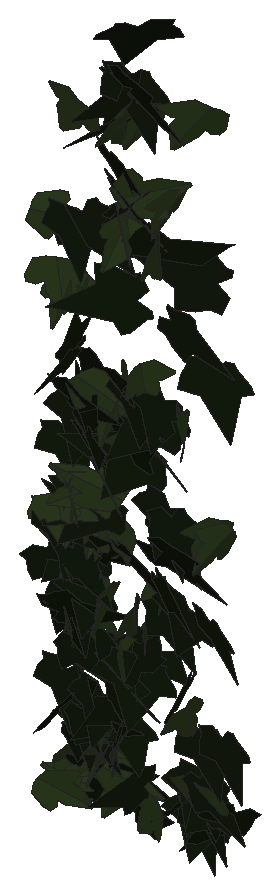
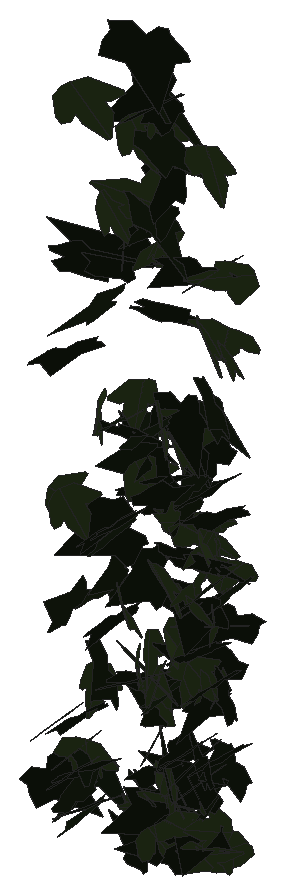
# SketchUp Ruby script. Lengths in inches.
U = 1.inch
M = Sketchup.active_model
def pt(a) = Geom::Point3d.new(a.map { |v| v * U })
def face(e, loops, mat)
  f = e.add_face(loops[0].map { |a| pt(a) })
  loops[1..].each { |l| e.add_face(l.map { |a| pt(a) }).erase! }
  f.material = f.back_material = mat if mat
  f
end
# faces: each face lists its corners as indices into pts; further lists are holes
def faces(e, pts, list, mat = nil) = list.each { |f| face(e, (f[0].is_a?(Array) ? f : [f]).map { |l| l.map { |i| pts[i] } }, mat) }
# xy, xz, yz: faces in a plane at the given z, y or x. An outline is a flat list of corners, or four numbers for a rectangle; further outlines are holes
def ring(l) = l.size == 4 ? [[l[0], l[1]], [l[2], l[1]], [l[2], l[3]], [l[0], l[3]]] : l.each_slice(2).to_a
def flat(e, list, mat, &to3) = list.each { |f| face(e, (f[0].is_a?(Array) ? f : [f]).map { |l| ring(l).map { |u, v| to3.(u, v) } }, mat) }
def xy(e, z, list, mat = nil) = flat(e, list, mat) { |x, y| [x, y, z] }
def xz(e, y, list, mat = nil) = flat(e, list, mat) { |x, z| [x, y, z] }
def yz(e, x, list, mat = nil) = flat(e, list, mat) { |y, z| [x, y, z] }
def lines(e, pts, list) = list.each { |a, b| e.add_line(pt(pts[a]), pt(pts[b])) }
# prism: a flat outline (further loops are holes) pulled along v
def prism(e, loops, v, mat = nil)
  f = face(e, loops, mat); d = Geom::Vector3d.new(v.map { |x| x * U })
  f.pushpull(f.normal.samedirection?(d) ? d.length : -d.length)
end
def box(e, o, s, mat = nil) = prism(e, [[o, [o[0] + s[0], o[1], o[2]], [o[0] + s[0], o[1] + s[1], o[2]], [o[0], o[1] + s[1], o[2]]]], [0, 0, s[2]], mat)
def at(x, y, z, deg = 0) = Geom::Transformation.translation(pt([x, y, z])) * Geom::Transformation.rotation(ORIGIN, Z_AXIS, deg.degrees)
def axes(o, x, y, z) = Geom::Transformation.new([*x, 0, *y, 0, *z, 0, *pt(o).to_a, 1])
def part(name) = M.definitions.add(name)
# library, detail: a bought-in or finely detailed component or shape, given as its bounding box
def library(name, o, s) = part(name).tap { |d| box(d.entities, o, s) }
def detail(e, o, s) = box(e.add_group.entities, o, s)
def put(e, d, t, mat = nil) = e.add_instance(d, t).tap { |i| i.material = mat if mat }
def group(e, t, mat = nil) = e.add_group.tap { |g| g.transformation = t; g.material = mat if mat }.entities
root = M.entities
M.materials.add("1026 AP 7946 SUNNY SIDE UP").color = [254, 231, 186]
M.materials.add("efeu1").color = [18, 25, 13]
M.materials.add("efeu2").color = [43, 57, 29]
c1 = part("ivyleaf_9")
p = [[1.54,2.16,1.25],[1.36,2.04,1.19],[-0.21,0.99,0.68],[-0.71,1.11,0.82],[-0.85,0.86,0.67],[-0.8,0.17,0.21],
  [-0.9,-0.01,0.1],[-0.67,-0.16,-0.02],[-0.08,-0.08,-0.05],[-0.03,-0.6,-0.4],[0.65,-0.88,-0.66],[0.83,-0.6,-0.49],
  [1.29,-0.42,-0.43],[1.8125,-0.07,-0.26],[1.21,0.44,0.15]]
faces(c1.entities,p,[[0,1,2,3,4,5,6,7,8,9,10,11,12,13,14]],"efeu1")
c2 = part("ivyleaf_10")
p = [[0,0.5,-0.03],[-0.0625,2.02,-0.43],[-0.19,2.01,-0.46],[-0.54,1.05,-0.29],[-0.52,0.625,-0.18],[-0.83,0.76,-0.28],
  [-1.16,0.64,-0.33],[-1.15,0.33,-0.24],[-0.77,-0.39,0.02],[-0.3,-0.51,0.16],[0.04,-0.48,0.23],[-0.02,2.01,-0.4375],
  [-0.06,2.01,-0.43],[0.04,-0.49,0.23],[0.67,-0.49,0.14],[1.38,0.36,-0.2],[1.375,0.51,-0.24],[0.81,0.65,-0.19],
  [0.62,0.59,-0.15],[0.6,1.09,-0.28],[0.5,1.23,-0.31]]
faces(c2.entities,p,[[0,1,2,3,4,5,6,7,8,9,10],[11,12,0,13,14,15,16,17,18,19,20]],"efeu2")
put(root,c1,axes([98.92,212.57,271.74],[0.07867,-0.26542,0.05597],[0.00956,-0.05567,-0.27854],[0.42638,0.05022,-0.00408]),"1026 AP 7946 SUNNY SIDE UP")
put(root,c1,axes([98.86,212.73,270.37],[0.00768,-0.04283,-0.2465],[0.3907,-0.03878,0.01205],[-0.06836,-0.22644,0.0412]),"1026 AP 7946 SUNNY SIDE UP")
put(root,c1,axes([99,212.74,269.39],[-0.03645,-0.26385,0.03472],[0.00036,-0.03535,-0.27305],[0.41855,-0.02295,0.00326]),"1026 AP 7946 SUNNY SIDE UP")
put(root,c2,axes([99.3125,212.57,277.98],[-0.37981,0.0743,0.14082],[-0.22478,0.01308,-0.25071],[-0.12044,-0.25872,0.02385]),"1026 AP 7946 SUNNY SIDE UP")
put(root,c1,axes([98.98,212.42,271.33],[-0.01322,-0.0951,-0.23583],[0.03641,0.21799,-0.0991],[0.40373,-0.02277,0.00122]),"1026 AP 7946 SUNNY SIDE UP")
put(root,c2,axes([98.875,212.42,276.33],[-0.04788,-0.07198,-0.2635],[0.37477,0.11735,-0.06243],[0.21843,-0.21712,0.04937]),"1026 AP 7946 SUNNY SIDE UP")
put(root,c1,axes([99,212.88,270.51],[0.01475,-0.27299,0.01382],[-0.00066,-0.01499,-0.28148],[0.42989,0.00934,-0.00091]),"1026 AP 7946 SUNNY SIDE UP")
put(root,c2,axes([99.1,212.57,270.43],[-0.15573,0.20855,-0.03662],[0.01063,-0.03755,-0.24424],[-0.35937,-0.09148,0.00865]),"1026 AP 7946 SUNNY SIDE UP")
put(root,c1,axes([99.23,212.52,274.39],[0.03624,0.127,0.23148],[0.01277,0.21493,-0.13399],[-0.42306,0.01737,0.01579]),"1026 AP 7946 SUNNY SIDE UP")
put(root,c1,axes([99.18,212.2,269.04],[-0.11239,0.14177,-0.19948],[-0.14207,0.16857,0.16984],[0.37387,0.10667,0.00457]),"1026 AP 7946 SUNNY SIDE UP")
put(root,c1,axes([99.05,212.72,272.94],[-0.07188,-0.22594,-0.06483],[0.03407,0.05481,-0.24513],[0.39435,-0.04592,0.00936]),"1026 AP 7946 SUNNY SIDE UP")
put(root,c2,axes([99.03,212.49,275.49],[0.40704,0.0632,0.06254],[0.10403,-0.00744,-0.26451],[-0.10122,0.24649,-0.02035]),"1026 AP 7946 SUNNY SIDE UP")
put(root,c2,axes([99.1,212.5,275.24],[0.30867,-0.16116,0.08469],[0.08643,-0.06478,-0.2606],[0.29391,0.18831,-0.01231]),"1026 AP 7946 SUNNY SIDE UP")
put(root,c2,axes([99.14,212.65,271.32],[-0.04199,0.10192,-0.22427],[-0.01397,-0.21223,-0.11177],[-0.39724,-0.00331,0.02764]),"1026 AP 7946 SUNNY SIDE UP")
put(root,c2,axes([99.38,212.73,267.82],[0.08322,0.11882,0.19662],[-0.24675,-0.12093,0.12467],[0.27453,-0.14471,0.05245]),"1026 AP 7946 SUNNY SIDE UP")
put(root,c1,axes([99.24,212.87,271.3],[-0.32905,-0.15842,0.09008],[0.00645,-0.13898,-0.24755],[0.28514,-0.17967,0.10956]),"1026 AP 7946 SUNNY SIDE UP")
put(root,c1,axes([99.31,212.53,274.33],[-0.25359,0.14222,-0.14828],[0.14119,-0.11509,-0.22122],[-0.30842,-0.16963,0.02065]),"1026 AP 7946 SUNNY SIDE UP")
put(root,c2,axes([99.125,212.53,268.2],[0.03368,-0.07345,0.23194],[0.03077,0.21824,0.08013],[-0.38865,0.01091,0.02644]),"1026 AP 7946 SUNNY SIDE UP")
put(root,c1,axes([99.36,212.88,271.6],[-0.03499,-0.27639,0.02424],[-0.00437,0.0254,0.28576],[-0.43636,0.02191,-0.00481]),"1026 AP 7946 SUNNY SIDE UP")
put(root,c1,axes([99.14,212.89,273.28],[-0.08545,-0.26215,0.09747],[-0.01725,-0.09582,-0.27623],[0.43869,-0.05483,0.00812]),"1026 AP 7946 SUNNY SIDE UP")
put(root,c2,axes([99.11,212.41,272.04],[0.35837,0.11994,0.04029],[0.0667,0.0037,-0.25932],[-0.20188,0.21414,-0.01416]),"1026 AP 7946 SUNNY SIDE UP")
put(root,c2,axes([99.06,212.31,267.91],[0.14805,0.09457,0.22014],[0.16656,0.18134,-0.13211],[-0.34412,0.12846,0.03076]),"1026 AP 7946 SUNNY SIDE UP")
put(root,c2,axes([99.15,212.54,267.93],[-0.1139,-0.11677,-0.19195],[0.19081,0.13878,-0.14107],[0.30651,-0.12979,0.01649]),"1026 AP 7946 SUNNY SIDE UP")
put(root,c2,axes([99.33,212.77,270.56],[-0.04162,-0.18797,0.12553],[-0.01659,-0.1194,-0.20454],[0.37794,-0.02594,0.00485]),"1026 AP 7946 SUNNY SIDE UP")
put(root,c2,axes([99.29,212.63,272.46],[0.08752,-0.21726,0.08136],[0.03333,-0.07636,-0.24011],[0.39091,0.05515,0.00226]),"1026 AP 7946 SUNNY SIDE UP")
put(root,c1,axes([99.47,212.72,272.12],[-0.36186,-0.07658,0.07247],[-0.08933,-0.05464,-0.24079],[0.15006,-0.21719,0.03142]),"1026 AP 7946 SUNNY SIDE UP")
put(root,c1,axes([99.16,212.8,269.08],[-0.02107,0.07026,0.23407],[0.0508,-0.21567,0.07333],[0.38503,0.0323,0.00313]),"1026 AP 7946 SUNNY SIDE UP")
put(root,c2,axes([99.26,212.49,272.22],[-0.15565,0.21968,-0.04486],[0.01506,-0.04478,-0.25529],[-0.38028,-0.09169,0.00825]),"1026 AP 7946 SUNNY SIDE UP")
put(root,c2,axes([99.36,212.56,275.41],[0.24966,-0.21134,-0.03509],[-0.03837,0.02083,-0.27527],[0.36032,0.14865,-0.005]),"1026 AP 7946 SUNNY SIDE UP")
put(root,c1,axes([99.21,212.56,268.68],[0.25063,-0.15497,-0.12351],[-0.13651,0.07993,-0.22801],[0.29595,0.1681,-0.00057]),"1026 AP 7946 SUNNY SIDE UP")
put(root,c2,axes([99.33,212.66,272.34],[0.06516,0.18271,-0.15873],[-0.04183,-0.1487,-0.20188],[-0.3998,0.04534,-0.00475]),"1026 AP 7946 SUNNY SIDE UP")
put(root,c1,axes([99.28,212.56,270.07],[0.05915,-0.14534,-0.19283],[-0.10046,0.16852,-0.15716],[0.37724,0.06767,-0.01162]),"1026 AP 7946 SUNNY SIDE UP")
put(root,c1,axes([99.36,212.64,268.24],[0.2761,0.14314,-0.04618],[-0.04147,-0.04022,-0.23205],[-0.25132,0.16389,-0.01245]),"1026 AP 7946 SUNNY SIDE UP")
put(root,c2,axes([99.41,212.72,270.45],[-0.35828,0.08586,-0.01357],[0.00713,-0.02609,-0.2431],[-0.14745,-0.20989,0.02121]),"1026 AP 7946 SUNNY SIDE UP")
put(root,c1,axes([99.39,212.65,271.53],[0.34596,0.06539,-0.11656],[-0.16857,-0.04885,-0.2293],[-0.13639,0.22625,-0.01225]),"1026 AP 7946 SUNNY SIDE UP")
put(root,c1,axes([99.27,212.53,276.28],[-0.00853,-0.26095,0.05202],[-0.00284,-0.05197,-0.28015],[0.45168,-0.00526,-0.00078]),"1026 AP 7946 SUNNY SIDE UP")
put(root,c2,axes([99.4,212.76,271.79],[0.06635,0.20411,-0.11197],[-0.02304,-0.10656,-0.22389],[-0.39073,0.04094,-0.00581]),"1026 AP 7946 SUNNY SIDE UP")
put(root,c1,axes([99.125,212.48,270.4375],[0.12023,-0.02463,0.23688],[0.37192,-0.03536,-0.07967],[0.07008,0.22993,0.01644]),"1026 AP 7946 SUNNY SIDE UP")
put(root,c2,axes([99.62,212.5,272.43],[0.25774,0.04967,-0.19867],[-0.29969,-0.05926,-0.17185],[-0.13124,0.23285,0.00225]),"1026 AP 7946 SUNNY SIDE UP")
put(root,c1,axes([99.58,212.45,273.44],[0.03737,-0.01877,0.26658],[-0.04749,0.24846,0.02614],[-0.42165,-0.02965,0.02068]),"1026 AP 7946 SUNNY SIDE UP")
put(root,c1,axes([99.4,212.74,270.8],[-0.11738,-0.22047,0.04447],[-0.01217,-0.04428,-0.24789],[0.38158,-0.06923,0.00578]),"1026 AP 7946 SUNNY SIDE UP")
put(root,c1,axes([99.35,212.74,268.88],[-0.00569,-0.25383,0.07463],[-0.01414,-0.07373,-0.26183],[0.41544,-0.00599,-0.00789]),"1026 AP 7946 SUNNY SIDE UP")
put(root,c2,axes([99.42,212.78,271.57],[0.32671,-0.12396,0.06229],[0.06339,-0.05192,-0.24461],[0.22488,0.19474,-0.02155]),"1026 AP 7946 SUNNY SIDE UP")
put(root,c1,axes([99.21,212.5625,273.6],[0.10105,-0.09816,0.22843],[0.24212,-0.16142,-0.12363],[0.31924,0.1535,0.02145]),"1026 AP 7946 SUNNY SIDE UP")
put(root,c2,axes([99.63,212.87,268.29],[0.16719,0.09065,-0.17735],[-0.22024,-0.1051,-0.1446],[-0.23533,0.16276,0.00933]),"1026 AP 7946 SUNNY SIDE UP")
put(root,c2,axes([99.77,212.44,268.7],[-0.00962,0.07765,0.26717],[-0.36099,0.13518,-0.04656],[-0.22431,-0.22088,0.06348]),"1026 AP 7946 SUNNY SIDE UP")
put(root,c1,axes([99.39,212.43,271.44],[0.13293,-0.20731,-0.11099],[-0.03434,0.10004,-0.23531],[0.38993,0.07949,0.01711]),"1026 AP 7946 SUNNY SIDE UP")
put(root,c1,axes([99.72,212.59,274.22],[0.23394,0.05972,-0.24471],[-0.37199,-0.03843,-0.1626],[-0.1017,0.27793,0.03183]),"1026 AP 7946 SUNNY SIDE UP")
put(root,c1,axes([99.69,212.66,272.15],[-0.396,-0.06236,-0.01193],[0.02663,-0.01885,-0.25768],[0.10394,-0.23275,0.02057]),"1026 AP 7946 SUNNY SIDE UP")
put(root,c1,axes([99.25,212.58,268.8125],[0.27155,0.05209,-0.17067],[0.2196,0.10331,0.17581],[0.18292,-0.20137,0.04231]),"1026 AP 7946 SUNNY SIDE UP")
put(root,c1,axes([99.43,212.72,273.15],[0.02367,-0.17536,0.18434],[0.02907,-0.17365,-0.19073],[0.41891,0.02196,0.00282]),"1026 AP 7946 SUNNY SIDE UP")
put(root,c2,axes([99.85,212.53,272.43],[0.12853,0.11597,0.25879],[-0.33068,-0.14314,0.1381],[0.28126,-0.22128,0.0441]),"1026 AP 7946 SUNNY SIDE UP")
put(root,c1,axes([99.38,212.66,273.07],[0.2387,-0.19472,0.04894],[0.03187,-0.0459,-0.25748],[0.33904,0.1414,-0.01026]),"1026 AP 7946 SUNNY SIDE UP")
put(root,c2,axes([99.59,212.76,270.91],[-0.02715,0.16293,-0.16991],[-0.01567,-0.16155,-0.17649],[-0.38832,-0.00487,0.019]),"1026 AP 7946 SUNNY SIDE UP")
put(root,c1,axes([99.39,212.62,276.37],[-0.04294,-0.16841,-0.21491],[0.21131,0.16738,-0.16663],[0.38816,-0.10975,0.06694]),"1026 AP 7946 SUNNY SIDE UP")
put(root,c1,axes([99.52,212.45,269.09],[0.18236,-0.22883,-0.12208],[-0.08117,0.10523,-0.26367],[0.39603,0.12694,0.00217]),"1026 AP 7946 SUNNY SIDE UP")
put(root,c1,axes([99.6,212.72,269.23],[-0.07488,-0.23828,0.11037],[-0.01723,-0.10836,-0.25077],[0.41132,-0.04792,0.00959]),"1026 AP 7946 SUNNY SIDE UP")
put(root,c1,axes([99.98,212.86,272.83],[-0.1409,0.02653,0.27677],[-0.37194,-0.14383,-0.06752],[0.2041,-0.2438,0.06801]),"1026 AP 7946 SUNNY SIDE UP")
put(root,c2,axes([99.76,212.51,268.54],[0.17418,-0.20811,0.04562],[0.01515,-0.04606,-0.24871],[0.36124,0.10227,-0.01157]),"1026 AP 7946 SUNNY SIDE UP")
put(root,c2,axes([99.81,212.56,268.76],[-0.08414,-0.2471,-0.08039],[0.03443,0.07365,-0.25997],[0.40533,-0.05755,0.0054]),"1026 AP 7946 SUNNY SIDE UP")
put(root,c2,axes([99.59,212.84,268.62],[0.09554,-0.03051,0.22885],[0.2787,-0.13806,-0.06917],[0.23911,0.17312,-0.01081]),"1026 AP 7946 SUNNY SIDE UP")
put(root,c2,axes([99.5625,212.51,273.96],[-0.22573,-0.07369,-0.21946],[0.36452,-0.01078,-0.14581],[0.05222,-0.2433,0.06922]),"1026 AP 7946 SUNNY SIDE UP")
put(root,c2,axes([99.79,212.69,270.875],[0.10027,-0.2264,0.14451],[0.06539,-0.13534,-0.24308],[0.41472,0.07608,0.00339]),"1026 AP 7946 SUNNY SIDE UP")
put(root,c2,axes([99.91,212.87,267.99],[-0.19464,-0.1827,0.1427],[-0.04276,-0.14575,-0.22228],[0.35896,-0.11643,0.0509]),"1026 AP 7946 SUNNY SIDE UP")
put(root,c1,axes([99.85,212.625,269.13],[-0.01713,-0.07159,-0.23594],[0.14787,-0.2046,0.06431],[-0.36288,-0.07999,0.03735]),"1026 AP 7946 SUNNY SIDE UP")
put(root,c1,axes([99.58,212.67,267.84],[0.26875,0.03587,0.15508],[0.2479,0.00285,-0.17214],[-0.0483,0.21425,-0.0206]),"1026 AP 7946 SUNNY SIDE UP")
put(root,c2,axes([99.77,212.63,273.67],[0.29612,-0.15742,0.10049],[0.10546,-0.07413,-0.25223],[0.29462,0.18476,-0.01072]),"1026 AP 7946 SUNNY SIDE UP")
put(root,c2,axes([99.96,212.73,271.76],[0.27206,-0.16362,-0.09706],[-0.11532,0.05731,-0.24426],[0.29399,0.17389,-0.00599]),"1026 AP 7946 SUNNY SIDE UP")
put(root,c2,axes([99.99,212.67,274.05],[0.06652,-0.18508,-0.19488],[-0.08012,0.17347,-0.19996],[0.43042,0.0609,-0.0071]),"1026 AP 7946 SUNNY SIDE UP")
put(root,c1,axes([99.92,212.52,269.6875],[0.19757,-0.04406,-0.24518],[-0.26982,0.17252,-0.12535],[0.26786,0.20627,0.05457]),"1026 AP 7946 SUNNY SIDE UP")
put(root,c1,axes([100.14,212.69,278.09],[-0.33011,0.15292,-0.15891],[0.05108,-0.19105,-0.24044],[-0.33867,-0.17787,0.11862]),"1026 AP 7946 SUNNY SIDE UP")
put(root,c1,axes([99.77,212.56,272.52],[0.01202,-0.09742,0.24306],[0.06286,-0.22543,-0.10736],[0.41665,0.03682,0.00918]),"1026 AP 7946 SUNNY SIDE UP")
put(root,c1,axes([100.27,212.53,275.43],[-0.39709,0.00751,0.15222],[-0.22941,-0.06065,-0.25414],[0.03819,-0.28621,0.0561]),"1026 AP 7946 SUNNY SIDE UP")
put(root,c1,axes([99.86,212.61,268.59],[0.01914,0.12357,0.23174],[-0.05452,-0.21253,0.1297],[0.41719,-0.03344,0.00632]),"1026 AP 7946 SUNNY SIDE UP")
put(root,c2,axes([99.92,212.68,268.6],[-0.02991,-0.08234,-0.24897],[0.01515,-0.23214,0.08443],[-0.4168,-0.00253,0.02093]),"1026 AP 7946 SUNNY SIDE UP")
put(root,c1,axes([99.79,212.74,270.09],[0.13055,-0.25735,-0.00117],[0.00696,0.00109,-0.27853],[0.4046,0.08302,0.00517]),"1026 AP 7946 SUNNY SIDE UP")
put(root,c1,axes([100.24,212.4,278.54],[-0.32522,0.22482,-0.04757],[0.03271,-0.04573,-0.31647],[-0.38865,-0.19198,0.01317]),"1026 AP 7946 SUNNY SIDE UP")
put(root,c1,axes([99.98,212.45,277.5],[0.38042,-0.08291,-0.16412],[-0.25847,0.02473,-0.25406],[0.14061,0.26978,-0.023]),"1026 AP 7946 SUNNY SIDE UP")
put(root,c1,axes([100.27,212.53,276.9],[-0.14175,0.27392,0.01619],[-0.03204,0.0063,-0.30599],[-0.46429,-0.08406,0.01618]),"1026 AP 7946 SUNNY SIDE UP")
put(root,c1,axes([99.96,212.78,268.94],[-0.04587,-0.21383,-0.06935],[0.01746,0.06118,-0.22988],[0.37753,-0.02881,0.00221]),"1026 AP 7946 SUNNY SIDE UP")
put(root,c2,axes([100.14,212.86,273.22],[-0.13263,-0.25362,0.10349],[-0.00689,-0.10537,-0.27454],[0.42972,-0.07997,0.02754]),"1026 AP 7946 SUNNY SIDE UP")
put(root,c2,axes([100.1,212.57,276.42],[0.15988,0.20295,-0.1901],[-0.11219,-0.16787,-0.2417],[-0.44687,0.11475,-0.00733]),"1026 AP 7946 SUNNY SIDE UP")
put(root,c2,axes([100.12,212.7,270.69],[0.04281,-0.25201,-0.1086],[0.03465,0.10619,-0.25858],[0.42727,0.01664,0.03185]),"1026 AP 7946 SUNNY SIDE UP")
put(root,c2,axes([100.17,212.4,278.14],[-0.06134,-0.25946,-0.14658],[0.02257,0.13295,-0.27855],[0.49483,-0.03823,-0.00546]),"1026 AP 7946 SUNNY SIDE UP")
put(root,c2,axes([99.84,212.73,269.875],[0.03712,-0.02386,0.28811],[0.40498,-0.11007,-0.0327],[0.17598,0.25833,0.01448]),"1026 AP 7946 SUNNY SIDE UP")
put(root,c2,axes([100.09,212.52,276.63],[-0.12335,0.27138,-0.06192],[0.00378,-0.06287,-0.30128],[-0.4723,-0.07138,0.01376]),"1026 AP 7946 SUNNY SIDE UP")
put(root,c1,axes([100.2,212.81,273],[-0.26739,-0.2032,0.10687],[-0.05749,-0.10487,-0.27097],[0.35494,-0.17006,0.03662]),"1026 AP 7946 SUNNY SIDE UP")
put(root,c1,axes([99.92,212.65,268.23],[0.35418,0.05068,0.0876],[0.14244,-0.0033,-0.22875],[-0.07808,0.22385,-0.01992]),"1026 AP 7946 SUNNY SIDE UP")
put(root,c2,axes([100.15,212.52,270.15],[-0.06553,0.26543,0.05948],[-0.04897,0.05183,-0.27554],[-0.42381,-0.04703,0.02264]),"1026 AP 7946 SUNNY SIDE UP")
put(root,c1,axes([100.26,212.64,279.43],[0.15201,0.25867,-0.11154],[-0.04072,-0.10543,-0.29429],[-0.47381,0.09205,-0.01049]),"1026 AP 7946 SUNNY SIDE UP")
put(root,c1,axes([100,212.53,277.02],[0.40376,-0.15898,-0.08649],[-0.11286,0.04183,-0.31087],[0.25846,0.26661,-0.00064]),"1026 AP 7946 SUNNY SIDE UP")
put(root,c2,axes([99.94,212.58,268.28],[-0.14718,-0.06308,-0.21662],[0.35603,-0.00039,-0.09648],[0.04169,-0.21938,0.05915]),"1026 AP 7946 SUNNY SIDE UP")
put(root,c2,axes([100.3125,212.76,278.16],[-0.15767,-0.25442,0.0943],[-0.0383,-0.08901,-0.29105],[0.45732,-0.09517,0.00814]),"1026 AP 7946 SUNNY SIDE UP")
put(root,c1,axes([100.48,212.41,270.08],[-0.05498,0.18634,0.20957],[-0.19177,0.17235,-0.18419],[-0.38772,-0.11167,0.06138]),"1026 AP 7946 SUNNY SIDE UP")
put(root,c1,axes([100.07,212.79,278.53],[0.01234,-0.30457,-0.00528],[0.04285,0.00408,-0.31257],[0.47701,0.00751,0.02821]),"1026 AP 7946 SUNNY SIDE UP")
put(root,c1,axes([100.1,212.82,273.77],[-0.03553,-0.22978,0.1761],[0.05448,-0.17369,-0.23505],[0.44825,0.0029,0.04253]),"1026 AP 7946 SUNNY SIDE UP")
put(root,c1,axes([99.97,212.55,269.72],[0.15003,-0.16993,0.19438],[0.17213,-0.15548,-0.20117],[0.36151,0.14455,0.01511]),"1026 AP 7946 SUNNY SIDE UP")
put(root,c1,axes([100.08,212.69,273.14],[-0.03833,0.03311,0.27169],[0.17764,-0.23083,0.03905],[0.39568,0.10684,0.00878]),"1026 AP 7946 SUNNY SIDE UP")
put(root,c1,axes([100.53,212.38,268.36],[-0.31779,0.18399,-0.01238],[-0.00387,-0.02219,-0.28071],[-0.31321,-0.18641,0.01603]),"1026 AP 7946 SUNNY SIDE UP")
put(root,c1,axes([100.01,212.54,278.64],[0.46616,-0.10509,0.03984],[0.03725,-0.04981,-0.32186],[0.17243,0.29488,-0.03818]),"1026 AP 7946 SUNNY SIDE UP")
put(root,c1,axes([100.08,212.86,267.61],[0.02759,-0.02071,0.23013],[0.18303,-0.18631,-0.03051],[0.31816,0.10898,-0.00241]),"1026 AP 7946 SUNNY SIDE UP")
put(root,c1,axes([100.11,212.56,271.625],[0.41227,-0.11674,-0.02025],[-0.04377,-0.01603,-0.29455],[0.18074,0.26239,-0.02516]),"1026 AP 7946 SUNNY SIDE UP")
put(root,c2,axes([100.33,212.67,274.29],[0.12051,0.25503,0.06627],[-0.09088,0.07357,-0.27241],[-0.4348,0.05531,0.07531]),"1026 AP 7946 SUNNY SIDE UP")
put(root,c2,axes([100.19,212.86,270.34],[0.14397,-0.14492,0.17877],[0.20097,-0.12364,-0.17897],[0.31987,0.14291,0.03199]),"1026 AP 7946 SUNNY SIDE UP")
put(root,c1,axes([100.55,212.74,273.66],[-0.43478,-0.05662,-0.00391],[0.01985,-0.03955,-0.2779],[0.09418,-0.25307,0.04051]),"1026 AP 7946 SUNNY SIDE UP")
put(root,c1,axes([100.4,212.91,270.09],[-0.20423,-0.22032,0.08655],[0.02176,-0.10424,-0.25635],[0.37083,-0.11522,0.06271]),"1026 AP 7946 SUNNY SIDE UP")
put(root,c1,axes([100.18,212.75,273.41],[0.30331,-0.18574,0.04801],[0.03165,-0.04746,-0.27582],[0.32381,0.17862,-0.01801]),"1026 AP 7946 SUNNY SIDE UP")
put(root,c1,axes([100.42,212.51,270.02],[-0.24812,-0.22254,-0.04316],[0.05724,0.02391,-0.28044],[0.35107,-0.16118,0.01522]),"1026 AP 7946 SUNNY SIDE UP")
put(root,c2,axes([100.28,212.51,276.97],[-0.1408,-0.0934,0.27928],[0.21882,0.22946,0.13443],[-0.41856,0.15138,-0.02367]),"1026 AP 7946 SUNNY SIDE UP")
put(root,c2,axes([100.45,212.81,271.12],[0.26025,-0.14712,0.14712],[0.15579,-0.10536,-0.22868],[0.30668,0.17837,-0.00868]),"1026 AP 7946 SUNNY SIDE UP")
put(root,c2,axes([100.63,212.48,268.02],[0.28296,-0.15895,-0.11151],[-0.08405,0.09979,-0.24398],[0.28964,0.18425,0.03814]),"1026 AP 7946 SUNNY SIDE UP")
put(root,c1,axes([100.49,212.87,273.86],[-0.11476,-0.24673,0.13171],[0.01167,-0.13529,-0.26253],[0.43782,-0.06107,0.04152]),"1026 AP 7946 SUNNY SIDE UP")
put(root,c2,axes([100.69,212.84,276.96],[-0.00926,-0.28198,0.10198],[-0.0013,-0.10059,-0.29114],[0.47074,-0.00583,0.0012]),"1026 AP 7946 SUNNY SIDE UP")
put(root,c1,axes([100.59,212.85,272.3],[-0.09899,-0.2245,0.10614],[-0.0352,-0.10004,-0.24966],[0.41714,-0.06172,0.00412]),"1026 AP 7946 SUNNY SIDE UP")
put(root,c1,axes([100.61,212.84,272.125],[0.05036,-0.24565,0.0793],[0.00833,-0.07723,-0.26594],[0.43707,0.02977,-0.00407]),"1026 AP 7946 SUNNY SIDE UP")
put(root,c2,axes([100.77,212.34,276.45],[0.09299,-0.27131,-0.11844],[0.05887,0.12171,-0.27907],[0.45863,0.03939,0.05984]),"1026 AP 7946 SUNNY SIDE UP")
put(root,c1,axes([100.66,212.76,270.89],[0.08112,-0.25222,-0.09926],[-0.04123,0.09148,-0.26458],[0.42173,0.05746,-0.00678]),"1026 AP 7946 SUNNY SIDE UP")
put(root,c1,axes([100.51,212.66,276.0625],[-0.00642,0.01866,0.30213],[0.4788,-0.01701,0.00502],[0.02936,0.28148,-0.01576]),"1026 AP 7946 SUNNY SIDE UP")
put(root,c1,axes([100.72,212.8,272.2],[0.07778,-0.26771,-0.07096],[-0.01176,0.06711,-0.28003],[0.43391,0.04981,0.00513]),"1026 AP 7946 SUNNY SIDE UP")
put(root,c1,axes([100.78,212.47,271.44],[0.29699,-0.19535,-0.06381],[-0.09495,0.02587,-0.27861],[0.30738,0.19674,-0.02441]),"1026 AP 7946 SUNNY SIDE UP")
put(root,c2,axes([101.08,212.53,273.6875],[0.02297,-0.00634,-0.30621],[-0.07423,0.29373,-0.00713],[0.4615,0.04756,0.01409]),"1026 AP 7946 SUNNY SIDE UP")
put(root,c1,axes([101.35,212.84,275.9375],[-0.25461,-0.1619,-0.1974],[-0.20516,-0.13915,0.23503],[-0.3356,0.2079,0.00609]),"1026 AP 7946 SUNNY SIDE UP")
put(root,c2,axes([101.18,212.85,278.375],[-0.26202,-0.21035,0.14993],[-0.11853,-0.12709,-0.27662],[0.38547,-0.18207,0.01686]),"1026 AP 7946 SUNNY SIDE UP")
put(root,c1,axes([101.12,212.34,269.76],[0.02095,0.15159,0.26331],[0.06906,0.25117,-0.15488],[-0.46096,0.04452,-0.01124]),"1026 AP 7946 SUNNY SIDE UP")
put(root,c1,axes([100.78,212.39,271.98],[0.46136,-0.02781,0.05359],[0.07764,-0.03,-0.30272],[0.05113,0.2965,-0.02384]),"1026 AP 7946 SUNNY SIDE UP")
put(root,c1,axes([101.29,212.43,268.45],[-0.18133,0.22298,-0.07913],[0.01429,-0.08263,-0.25742],[-0.37121,-0.1121,0.02874]),"1026 AP 7946 SUNNY SIDE UP")
put(root,c1,axes([100.93,212.56,275.31],[0.31094,-0.18082,-0.12167],[-0.04707,0.13432,-0.26501],[0.33543,0.18646,0.0756]),"1026 AP 7946 SUNNY SIDE UP")
put(root,c1,axes([101.0625,212.69,271.01],[-0.11079,-0.21834,0.15364],[0.02469,-0.15877,-0.23082],[0.41614,-0.04871,0.0546]),"1026 AP 7946 SUNNY SIDE UP")
put(root,c1,axes([101.13,212.88,267.98],[-0.13807,-0.22869,0.07859],[0.02151,-0.08713,-0.24914],[0.37911,-0.07834,0.04275]),"1026 AP 7946 SUNNY SIDE UP")
put(root,c1,axes([101.07,212.9,267.9],[0.06453,-0.24709,0.05296],[0.00578,-0.05292,-0.2583],[0.39726,0.04091,-0.00485]),"1026 AP 7946 SUNNY SIDE UP")
put(root,c2,axes([101.23,212.41,269.71],[-0.08001,-0.24298,-0.11131],[0.05959,0.10084,-0.25469],[0.41298,-0.06163,0.01518]),"1026 AP 7946 SUNNY SIDE UP")
put(root,c1,axes([101.22,212.8,268.47],[-0.15346,-0.23501,0.06746],[-0.00464,-0.07082,-0.26144],[0.38415,-0.09474,0.02379]),"1026 AP 7946 SUNNY SIDE UP")
put(root,c2,axes([101.4,212.47,268.56],[-0.40565,-0.00081,0.05129],[-0.07791,-0.02226,-0.26496],[0.00787,-0.2618,0.02083]),"1026 AP 7946 SUNNY SIDE UP")
put(root,c1,axes([101.17,212.92,268.125],[-0.00127,-0.18487,0.18596],[0.07937,-0.1782,-0.18773],[0.39963,0.03481,0.03788]),"1026 AP 7946 SUNNY SIDE UP")
put(root,c1,axes([101.18,212.89,268.09],[0.10944,-0.24252,0.05893],[0.01267,-0.0586,-0.26013],[0.3921,0.06958,-0.00804]),"1026 AP 7946 SUNNY SIDE UP")
put(root,c2,axes([101.43,212.79,272.34],[-0.1224,-0.2484,0.10735],[-0.00794,-0.10856,-0.2675],[0.42434,-0.07368,0.02596]),"1026 AP 7946 SUNNY SIDE UP")
put(root,c1,axes([101.28,212.73,269.21],[0.01119,-0.26812,-0.02344],[0.00939,0.02139,-0.2761],[0.4228,0.00662,0.00675]),"1026 AP 7946 SUNNY SIDE UP")
put(root,c1,axes([101.46,212.8,268.27],[-0.15193,-0.16402,0.18206],[-0.08,-0.17324,-0.19429],[0.37168,-0.10433,0.0326]),"1026 AP 7946 SUNNY SIDE UP")
put(root,c1,axes([101.37,212.875,274.6],[-0.05676,-0.28335,-0.06394],[0.02072,0.05925,-0.29386],[0.45509,-0.03804,0.0054]),"1026 AP 7946 SUNNY SIDE UP")
put(root,c1,axes([101.3,212.86,270.83],[0.14164,-0.23241,0.11657],[0.04714,-0.11103,-0.25718],[0.40463,0.09429,-0.01084]),"1026 AP 7946 SUNNY SIDE UP")
put(root,c1,axes([101.39,212.59,268.64],[0.18182,-0.23156,-0.09765],[-0.03541,0.09292,-0.26529],[0.39105,0.11608,0.02138]),"1026 AP 7946 SUNNY SIDE UP")
put(root,c2,axes([101.63,212.68,272.32],[-0.04507,-0.19135,0.21116],[0.01088,-0.20754,-0.19877],[0.44203,-0.0144,0.02642]),"1026 AP 7946 SUNNY SIDE UP")
put(root,c1,axes([101.76,212.73,268.24],[-0.05891,0.12063,-0.2388],[0.00549,-0.23461,-0.12735],[-0.41181,-0.02038,0.03246]),"1026 AP 7946 SUNNY SIDE UP")
put(root,c1,axes([101.47,212.88,269.16],[0.0672,-0.26357,0.00833],[0.00098,-0.0096,-0.27513],[0.41472,0.04273,-0.0007]),"1026 AP 7946 SUNNY SIDE UP")
